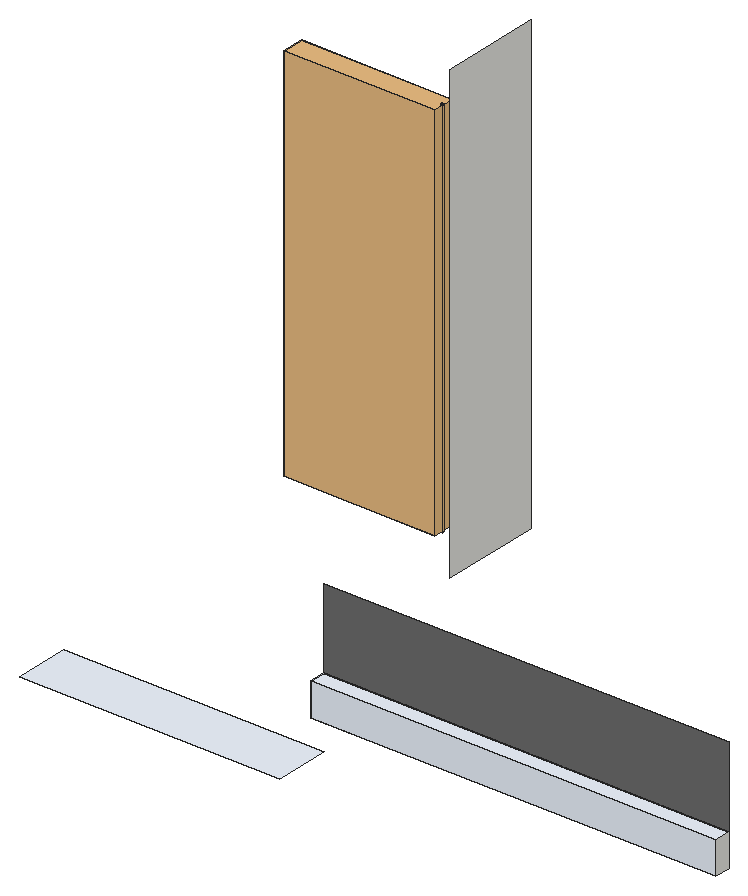
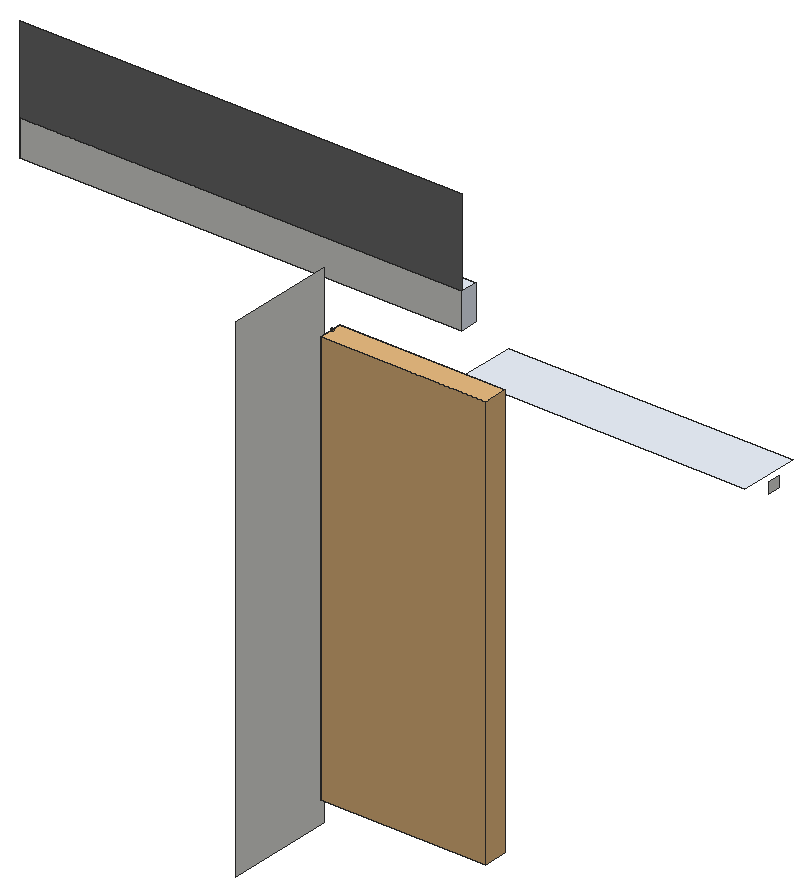
# SketchUp Ruby script. Lengths in inches.
U = 1.inch
M = Sketchup.active_model
def pt(a) = Geom::Point3d.new(a.map { |v| v * U })
def face(e, loops, mat)
  f = e.add_face(loops[0].map { |a| pt(a) })
  loops[1..].each { |l| e.add_face(l.map { |a| pt(a) }).erase! }
  f.material = f.back_material = mat if mat
  f
end
# faces: each face lists its corners as indices into pts; further lists are holes
def faces(e, pts, list, mat = nil) = list.each { |f| face(e, (f[0].is_a?(Array) ? f : [f]).map { |l| l.map { |i| pts[i] } }, mat) }
# xy, xz, yz: faces in a plane at the given z, y or x. An outline is a flat list of corners, or four numbers for a rectangle; further outlines are holes
def ring(l) = l.size == 4 ? [[l[0], l[1]], [l[2], l[1]], [l[2], l[3]], [l[0], l[3]]] : l.each_slice(2).to_a
def flat(e, list, mat, &to3) = list.each { |f| face(e, (f[0].is_a?(Array) ? f : [f]).map { |l| ring(l).map { |u, v| to3.(u, v) } }, mat) }
def xy(e, z, list, mat = nil) = flat(e, list, mat) { |x, y| [x, y, z] }
def xz(e, y, list, mat = nil) = flat(e, list, mat) { |x, z| [x, y, z] }
def yz(e, x, list, mat = nil) = flat(e, list, mat) { |y, z| [x, y, z] }
def lines(e, pts, list) = list.each { |a, b| e.add_line(pt(pts[a]), pt(pts[b])) }
# prism: a flat outline (further loops are holes) pulled along v
def prism(e, loops, v, mat = nil)
  f = face(e, loops, mat); d = Geom::Vector3d.new(v.map { |x| x * U })
  f.pushpull(f.normal.samedirection?(d) ? d.length : -d.length)
end
def box(e, o, s, mat = nil) = prism(e, [[o, [o[0] + s[0], o[1], o[2]], [o[0] + s[0], o[1] + s[1], o[2]], [o[0], o[1] + s[1], o[2]]]], [0, 0, s[2]], mat)
def at(x, y, z, deg = 0) = Geom::Transformation.translation(pt([x, y, z])) * Geom::Transformation.rotation(ORIGIN, Z_AXIS, deg.degrees)
def axes(o, x, y, z) = Geom::Transformation.new([*x, 0, *y, 0, *z, 0, *pt(o).to_a, 1])
def part(name) = M.definitions.add(name)
# library, detail: a bought-in or finely detailed component or shape, given as its bounding box
def library(name, o, s) = part(name).tap { |d| box(d.entities, o, s) }
def detail(e, o, s) = box(e.add_group.entities, o, s)
def put(e, d, t, mat = nil) = e.add_instance(d, t).tap { |i| i.material = mat if mat }
def group(e, t, mat = nil) = e.add_group.tap { |g| g.transformation = t; g.material = mat if mat }.entities
root = M.entities
M.materials.add("Generic").color = [111, 111, 111]
M.materials.add("Generic\#4").color = [238, 245, 255]
M.materials.add("Material \#1").color = [140, 140, 140]
c1 = library("3DGeom~6_Defintion",[-5.59,-471.8,-48.03],[468.87,1000,73.72])
c2 = library("3DGeom~9_Defintion",[456.52,-471.89,-18.89],[5.57,1000,5.49])
c3 = library("3DGeom~7_Defintion",[455.56,-471.94,-18.85],[5.55,1000,5.48])
c4 = part("3DGeom~8_Defintion")
xz(c4.entities,-471.94,[[458.125,-17.29,459.53,-16.11,457.73,-17.15],[458.125,-17.29,458.54,-17.29,459.53,-16.11],[458.54,-17.29,458.93,-17.15,459.53,-16.11],[457.73,-17.15,459.53,-16.11,457.42,-16.88],[458.93,-17.15,459.25,-16.88,459.53,-16.11],
  [457.42,-16.88,459.53,-16.11,457.21,-16.52],[459.25,-16.88,459.46,-16.52,459.53,-16.11],[457.21,-16.52,459.53,-16.11,457.14,-16.11],[457.14,-16.11,459.53,-16.11,457.21,-15.7],[459.53,-16.11,457.42,-15.34,457.21,-15.7],
  [459.53,-16.11,457.73,-15.07,457.42,-15.34],[459.53,-16.11,458.125,-14.93,457.73,-15.07],[459.53,-16.11,458.54,-14.93,458.125,-14.93],[459.53,-16.11,458.93,-15.07,458.54,-14.93],[459.53,-16.11,459.25,-15.34,458.93,-15.07],
  [459.53,-16.11,459.46,-15.7,459.25,-15.34]],"Material \#1")
xz(c4.entities,-416.39,[[458.125,-17.29,457.73,-17.15,459.53,-16.11],[458.125,-17.29,459.53,-16.11,458.54,-17.29],[458.54,-17.29,459.53,-16.11,458.93,-17.15],[457.73,-17.15,457.42,-16.88,459.53,-16.11],[458.93,-17.15,459.53,-16.11,459.25,-16.88],
  [457.42,-16.88,457.21,-16.52,459.53,-16.11],[459.25,-16.88,459.53,-16.11,459.46,-16.52],[457.21,-16.52,457.14,-16.11,459.53,-16.11],[457.14,-16.11,457.21,-15.7,459.53,-16.11],[459.53,-16.11,457.21,-15.7,457.42,-15.34],
  [459.53,-16.11,457.42,-15.34,457.73,-15.07],[459.53,-16.11,457.73,-15.07,458.125,-14.93],[459.53,-16.11,458.125,-14.93,458.54,-14.93],[459.53,-16.11,458.54,-14.93,458.93,-15.07],[459.53,-16.11,458.93,-15.07,459.25,-15.34],
  [459.53,-16.11,459.25,-15.34,459.46,-15.7]],"Material \#1")
xz(c4.entities,-27.5,[[458.125,-17.29,459.53,-16.11,457.73,-17.15],[458.125,-17.29,458.54,-17.29,459.53,-16.11],[458.54,-17.29,458.93,-17.15,459.53,-16.11],[457.73,-17.15,459.53,-16.11,457.42,-16.88],[458.93,-17.15,459.25,-16.88,459.53,-16.11],
  [457.42,-16.88,459.53,-16.11,457.21,-16.52],[459.25,-16.88,459.46,-16.52,459.53,-16.11],[457.21,-16.52,459.53,-16.11,457.14,-16.11],[457.14,-16.11,459.53,-16.11,457.21,-15.7],[459.53,-16.11,457.42,-15.34,457.21,-15.7],
  [459.53,-16.11,457.73,-15.07,457.42,-15.34],[459.53,-16.11,458.125,-14.93,457.73,-15.07],[459.53,-16.11,458.54,-14.93,458.125,-14.93],[459.53,-16.11,458.93,-15.07,458.54,-14.93],[459.53,-16.11,459.25,-15.34,458.93,-15.07],
  [459.53,-16.11,459.46,-15.7,459.25,-15.34]],"Material \#1")
xz(c4.entities,28.06,[[458.125,-17.29,457.73,-17.15,459.53,-16.11],[458.125,-17.29,459.53,-16.11,458.54,-17.29],[458.54,-17.29,459.53,-16.11,458.93,-17.15],[457.73,-17.15,457.42,-16.88,459.53,-16.11],[458.93,-17.15,459.53,-16.11,459.25,-16.88],
  [457.42,-16.88,457.21,-16.52,459.53,-16.11],[459.25,-16.88,459.53,-16.11,459.46,-16.52],[457.21,-16.52,457.14,-16.11,459.53,-16.11],[457.14,-16.11,457.21,-15.7,459.53,-16.11],[459.53,-16.11,457.21,-15.7,457.42,-15.34],
  [459.53,-16.11,457.42,-15.34,457.73,-15.07],[459.53,-16.11,457.73,-15.07,458.125,-14.93],[459.53,-16.11,458.125,-14.93,458.54,-14.93],[459.53,-16.11,458.54,-14.93,458.93,-15.07],[459.53,-16.11,458.93,-15.07,459.25,-15.34],
  [459.53,-16.11,459.25,-15.34,459.46,-15.7]],"Material \#1")
xz(c4.entities,472.5,[[458.125,-17.29,459.53,-16.11,457.73,-17.15],[458.125,-17.29,458.54,-17.29,459.53,-16.11],[458.54,-17.29,458.93,-17.15,459.53,-16.11],[457.73,-17.15,459.53,-16.11,457.42,-16.88],[458.93,-17.15,459.25,-16.88,459.53,-16.11],
  [457.42,-16.88,459.53,-16.11,457.21,-16.52],[459.25,-16.88,459.46,-16.52,459.53,-16.11],[457.21,-16.52,459.53,-16.11,457.14,-16.11],[457.14,-16.11,459.53,-16.11,457.21,-15.7],[459.53,-16.11,457.42,-15.34,457.21,-15.7],
  [459.53,-16.11,457.73,-15.07,457.42,-15.34],[459.53,-16.11,458.125,-14.93,457.73,-15.07],[459.53,-16.11,458.54,-14.93,458.125,-14.93],[459.53,-16.11,458.93,-15.07,458.54,-14.93],[459.53,-16.11,459.25,-15.34,458.93,-15.07],
  [459.53,-16.11,459.46,-15.7,459.25,-15.34]],"Material \#1")
xz(c4.entities,528.06,[[458.125,-17.29,457.73,-17.15,459.53,-16.11],[458.125,-17.29,459.53,-16.11,458.54,-17.29],[458.54,-17.29,459.53,-16.11,458.93,-17.15],[457.73,-17.15,457.42,-16.88,459.53,-16.11],[458.93,-17.15,459.53,-16.11,459.25,-16.88],
  [457.42,-16.88,457.21,-16.52,459.53,-16.11],[459.25,-16.88,459.53,-16.11,459.46,-16.52],[457.21,-16.52,457.14,-16.11,459.53,-16.11],[457.14,-16.11,457.21,-15.7,459.53,-16.11],[459.53,-16.11,457.21,-15.7,457.42,-15.34],
  [459.53,-16.11,457.42,-15.34,457.73,-15.07],[459.53,-16.11,457.73,-15.07,458.125,-14.93],[459.53,-16.11,458.125,-14.93,458.54,-14.93],[459.53,-16.11,458.54,-14.93,458.93,-15.07],[459.53,-16.11,458.93,-15.07,459.25,-15.34],
  [459.53,-16.11,459.25,-15.34,459.46,-15.7]],"Material \#1")
xy(root,162.6,[[128.43,116.3125,128.38,116.33,128.39,116.35],[128.43,116.3125,128.39,116.35,128.4375,116.33],[128.43,116.3125,128.4375,116.33,128.49,116.3125],[128.49,116.3125,128.4375,116.33,128.49,116.33],[128.49,116.3125,128.49,116.33,128.55,116.33],
  [128.38,116.33,128.34,116.37,128.35,116.375],[128.38,116.33,128.35,116.375,128.39,116.35],[128.49,116.33,128.54,116.35,128.55,116.33],[128.55,116.33,128.54,116.35,128.59,116.37],[128.54,116.35,128.58,116.375,128.59,116.37],
  [128.34,116.37,128.31,116.41,128.32,116.42],[128.34,116.37,128.32,116.42,128.35,116.375],[128.59,116.37,128.58,116.375,128.62,116.41],[128.58,116.375,128.6,116.42,128.62,116.41],[128.31,116.41,128.3,116.47,128.32,116.47],
  [128.31,116.41,128.32,116.47,128.32,116.42],[128.62,116.41,128.6,116.42,128.63,116.47],[128.6,116.42,128.61,116.47,128.63,116.47],[128.3,116.47,128.31,116.52,128.32,116.51],[128.3,116.47,128.32,116.51,128.32,116.47],
  [128.61,116.47,128.6,116.51,128.62,116.52],[128.61,116.47,128.62,116.52,128.63,116.47],[128.32,116.51,128.31,116.52,128.35,116.55],[128.6,116.51,128.58,116.55,128.59,116.5625],[128.6,116.51,128.59,116.5625,128.62,116.52],
  [128.31,116.52,128.34,116.5625,128.35,116.55],[128.35,116.55,128.34,116.5625,128.39,116.58],[128.58,116.55,128.54,116.58,128.55,116.6],[128.58,116.55,128.55,116.6,128.59,116.5625],[128.34,116.5625,128.38,116.6,128.39,116.58],
  [128.39,116.58,128.38,116.6,128.4375,116.6],[128.54,116.58,128.49,116.6,128.49,116.62],[128.54,116.58,128.49,116.62,128.55,116.6],[128.38,116.6,128.43,116.62,128.4375,116.6],[128.4375,116.6,128.43,116.62,128.49,116.6],
  [128.49,116.6,128.43,116.62,128.49,116.62]],"Material \#1")
xy(root,162.61,[[128.43,116.3125,128.4375,116.33,128.38,116.33],[128.43,116.3125,128.49,116.3125,128.49,116.33],[128.43,116.3125,128.49,116.33,128.4375,116.33],[128.49,116.3125,128.54,116.35,128.49,116.33],[128.49,116.3125,128.55,116.33,128.54,116.35],
  [128.38,116.33,128.39,116.35,128.34,116.37],[128.38,116.33,128.4375,116.33,128.39,116.35],[128.55,116.33,128.58,116.375,128.54,116.35],[128.55,116.33,128.59,116.37,128.58,116.375],[128.39,116.35,128.35,116.375,128.34,116.37],
  [128.34,116.37,128.35,116.375,128.31,116.41],[128.59,116.37,128.6,116.42,128.58,116.375],[128.59,116.37,128.62,116.41,128.6,116.42],[128.35,116.375,128.32,116.42,128.31,116.41],[128.31,116.41,128.32,116.42,128.3,116.47],
  [128.62,116.41,128.61,116.47,128.6,116.42],[128.62,116.41,128.63,116.47,128.61,116.47],[128.32,116.42,128.32,116.47,128.3,116.47],[128.3,116.47,128.32,116.47,128.31,116.52],[128.32,116.47,128.32,116.51,128.31,116.52],
  [128.61,116.47,128.63,116.47,128.6,116.51],[128.63,116.47,128.62,116.52,128.6,116.51],[128.32,116.51,128.34,116.5625,128.31,116.52],[128.32,116.51,128.35,116.55,128.34,116.5625],[128.6,116.51,128.62,116.52,128.58,116.55],
  [128.62,116.52,128.59,116.5625,128.58,116.55],[128.35,116.55,128.38,116.6,128.34,116.5625],[128.35,116.55,128.39,116.58,128.38,116.6],[128.58,116.55,128.59,116.5625,128.54,116.58],[128.59,116.5625,128.55,116.6,128.54,116.58],
  [128.39,116.58,128.43,116.62,128.38,116.6],[128.39,116.58,128.4375,116.6,128.43,116.62],[128.54,116.58,128.55,116.6,128.49,116.6],[128.4375,116.6,128.49,116.62,128.43,116.62],[128.4375,116.6,128.49,116.6,128.49,116.62],
  [128.49,116.6,128.55,116.6,128.49,116.62]],"Material \#1")
xy(root,166.09,[[128.43,116.3125,128.38,116.33,128.4375,116.33],[128.43,116.3125,128.4375,116.33,128.49,116.33],[128.43,116.3125,128.49,116.33,128.49,116.3125],[128.49,116.3125,128.49,116.33,128.54,116.35],[128.49,116.3125,128.54,116.35,128.55,116.33],
  [128.38,116.33,128.34,116.37,128.39,116.35],[128.38,116.33,128.39,116.35,128.4375,116.33],[128.55,116.33,128.54,116.35,128.58,116.375],[128.55,116.33,128.58,116.375,128.59,116.37],[128.39,116.35,128.34,116.37,128.35,116.375],
  [128.34,116.37,128.31,116.41,128.35,116.375],[128.59,116.37,128.58,116.375,128.6,116.42],[128.59,116.37,128.6,116.42,128.62,116.41],[128.35,116.375,128.31,116.41,128.32,116.42],[128.31,116.41,128.3,116.47,128.32,116.42],
  [128.62,116.41,128.6,116.42,128.61,116.47],[128.62,116.41,128.61,116.47,128.63,116.47],[128.32,116.42,128.3,116.47,128.32,116.47],[128.3,116.47,128.31,116.52,128.32,116.47],[128.32,116.47,128.31,116.52,128.32,116.51],
  [128.61,116.47,128.6,116.51,128.63,116.47],[128.63,116.47,128.6,116.51,128.62,116.52],[128.32,116.51,128.31,116.52,128.34,116.5625],[128.32,116.51,128.34,116.5625,128.35,116.55],[128.6,116.51,128.58,116.55,128.62,116.52],
  [128.62,116.52,128.58,116.55,128.59,116.5625],[128.35,116.55,128.34,116.5625,128.38,116.6],[128.35,116.55,128.38,116.6,128.39,116.58],[128.58,116.55,128.54,116.58,128.59,116.5625],[128.59,116.5625,128.54,116.58,128.55,116.6],
  [128.39,116.58,128.38,116.6,128.43,116.62],[128.39,116.58,128.43,116.62,128.4375,116.6],[128.54,116.58,128.49,116.6,128.55,116.6],[128.4375,116.6,128.43,116.62,128.49,116.62],[128.4375,116.6,128.49,116.62,128.49,116.6],
  [128.49,116.6,128.49,116.62,128.55,116.6]],"Material \#1")
xy(root,166.1,[[128.43,116.3125,128.39,116.35,128.38,116.33],[128.43,116.3125,128.4375,116.33,128.39,116.35],[128.43,116.3125,128.49,116.3125,128.4375,116.33],[128.49,116.3125,128.49,116.33,128.4375,116.33],[128.49,116.3125,128.55,116.33,128.49,116.33],
  [128.38,116.33,128.35,116.375,128.34,116.37],[128.38,116.33,128.39,116.35,128.35,116.375],[128.49,116.33,128.55,116.33,128.54,116.35],[128.55,116.33,128.59,116.37,128.54,116.35],[128.54,116.35,128.59,116.37,128.58,116.375],
  [128.34,116.37,128.32,116.42,128.31,116.41],[128.34,116.37,128.35,116.375,128.32,116.42],[128.59,116.37,128.62,116.41,128.58,116.375],[128.58,116.375,128.62,116.41,128.6,116.42],[128.31,116.41,128.32,116.47,128.3,116.47],
  [128.31,116.41,128.32,116.42,128.32,116.47],[128.62,116.41,128.63,116.47,128.6,116.42],[128.6,116.42,128.63,116.47,128.61,116.47],[128.3,116.47,128.32,116.47,128.32,116.51],[128.3,116.47,128.32,116.51,128.31,116.52],
  [128.61,116.47,128.62,116.52,128.6,116.51],[128.61,116.47,128.63,116.47,128.62,116.52],[128.32,116.51,128.35,116.55,128.31,116.52],[128.6,116.51,128.59,116.5625,128.58,116.55],[128.6,116.51,128.62,116.52,128.59,116.5625],
  [128.31,116.52,128.35,116.55,128.34,116.5625],[128.35,116.55,128.39,116.58,128.34,116.5625],[128.58,116.55,128.55,116.6,128.54,116.58],[128.58,116.55,128.59,116.5625,128.55,116.6],[128.34,116.5625,128.39,116.58,128.38,116.6],
  [128.39,116.58,128.4375,116.6,128.38,116.6],[128.54,116.58,128.49,116.62,128.49,116.6],[128.54,116.58,128.55,116.6,128.49,116.62],[128.38,116.6,128.4375,116.6,128.43,116.62],[128.4375,116.6,128.49,116.6,128.43,116.62],
  [128.49,116.6,128.49,116.62,128.43,116.62]],"Material \#1")
xy(root,175.6875,[[122.63,27.72,169.98,37.59]],"Generic\#4")
xy(root,182.625,[[169.98,34.65,243.69,37.59]],"Generic\#4")
xy(root,188.5625,[[169.98,34.65,243.69,37.59]],"Generic\#4")
xy(root,193.58,[[128.43,116.3125,128.38,116.33,128.39,116.35],[128.43,116.3125,128.39,116.35,128.4375,116.33],[128.43,116.3125,128.4375,116.33,128.49,116.3125],[128.49,116.3125,128.4375,116.33,128.49,116.33],[128.49,116.3125,128.49,116.33,128.55,116.33],
  [128.38,116.33,128.34,116.37,128.35,116.375],[128.38,116.33,128.35,116.375,128.39,116.35],[128.49,116.33,128.54,116.35,128.55,116.33],[128.55,116.33,128.54,116.35,128.59,116.37],[128.54,116.35,128.58,116.375,128.59,116.37],
  [128.34,116.37,128.31,116.41,128.32,116.42],[128.34,116.37,128.32,116.42,128.35,116.375],[128.59,116.37,128.58,116.375,128.62,116.41],[128.58,116.375,128.6,116.42,128.62,116.41],[128.31,116.41,128.3,116.47,128.32,116.47],
  [128.31,116.41,128.32,116.47,128.32,116.42],[128.62,116.41,128.6,116.42,128.63,116.47],[128.6,116.42,128.61,116.47,128.63,116.47],[128.3,116.47,128.31,116.52,128.32,116.51],[128.3,116.47,128.32,116.51,128.32,116.47],
  [128.61,116.47,128.6,116.51,128.62,116.52],[128.61,116.47,128.62,116.52,128.63,116.47],[128.32,116.51,128.31,116.52,128.35,116.55],[128.6,116.51,128.58,116.55,128.59,116.5625],[128.6,116.51,128.59,116.5625,128.62,116.52],
  [128.31,116.52,128.34,116.5625,128.35,116.55],[128.35,116.55,128.34,116.5625,128.39,116.58],[128.58,116.55,128.54,116.58,128.55,116.6],[128.58,116.55,128.55,116.6,128.59,116.5625],[128.34,116.5625,128.38,116.6,128.39,116.58],
  [128.39,116.58,128.38,116.6,128.4375,116.6],[128.54,116.58,128.49,116.6,128.49,116.62],[128.54,116.58,128.49,116.62,128.55,116.6],[128.38,116.6,128.43,116.62,128.4375,116.6],[128.4375,116.6,128.43,116.62,128.49,116.6],
  [128.49,116.6,128.43,116.62,128.49,116.62]],"Material \#1")
xy(root,193.6,[[128.43,116.3125,128.4375,116.33,128.38,116.33],[128.43,116.3125,128.49,116.3125,128.49,116.33],[128.43,116.3125,128.49,116.33,128.4375,116.33],[128.49,116.3125,128.54,116.35,128.49,116.33],[128.49,116.3125,128.55,116.33,128.54,116.35],
  [128.38,116.33,128.39,116.35,128.34,116.37],[128.38,116.33,128.4375,116.33,128.39,116.35],[128.55,116.33,128.58,116.375,128.54,116.35],[128.55,116.33,128.59,116.37,128.58,116.375],[128.39,116.35,128.35,116.375,128.34,116.37],
  [128.34,116.37,128.35,116.375,128.31,116.41],[128.59,116.37,128.6,116.42,128.58,116.375],[128.59,116.37,128.62,116.41,128.6,116.42],[128.35,116.375,128.32,116.42,128.31,116.41],[128.31,116.41,128.32,116.42,128.3,116.47],
  [128.62,116.41,128.61,116.47,128.6,116.42],[128.62,116.41,128.63,116.47,128.61,116.47],[128.32,116.42,128.32,116.47,128.3,116.47],[128.3,116.47,128.32,116.47,128.31,116.52],[128.32,116.47,128.32,116.51,128.31,116.52],
  [128.61,116.47,128.63,116.47,128.6,116.51],[128.63,116.47,128.62,116.52,128.6,116.51],[128.32,116.51,128.34,116.5625,128.31,116.52],[128.32,116.51,128.35,116.55,128.34,116.5625],[128.6,116.51,128.62,116.52,128.58,116.55],
  [128.62,116.52,128.59,116.5625,128.58,116.55],[128.35,116.55,128.38,116.6,128.34,116.5625],[128.35,116.55,128.39,116.58,128.38,116.6],[128.58,116.55,128.59,116.5625,128.54,116.58],[128.59,116.5625,128.55,116.6,128.54,116.58],
  [128.39,116.58,128.43,116.62,128.38,116.6],[128.39,116.58,128.4375,116.6,128.43,116.62],[128.54,116.58,128.55,116.6,128.49,116.6],[128.4375,116.6,128.49,116.62,128.43,116.62],[128.4375,116.6,128.49,116.6,128.49,116.62],
  [128.49,116.6,128.55,116.6,128.49,116.62]],"Material \#1")
xz(root,34.65,[[169.98,182.625,243.69,188.5625]],"Generic\#4")
xz(root,37.59,[[169.98,182.625,243.69,188.5625]])
xz(root,37.59,[[169.98,188.5625,243.69,203.1875]],"Generic")
yz(root,122.04,[[31.35,173.3125,33.48,175.125]])
yz(root,131.25,[[114.72,156.59,133.09,239.46]])
yz(root,169.98,[[34.65,182.625,37.59,188.5625]],"Generic\#4")
yz(root,243.69,[[34.65,182.625,37.59,188.5625]])
put(root,c1,axes([101.39,117.36,195.3125],[0.05875,0,0],[0,0,0.06934],[0,0.05495,0]),"Material \#1")
put(root,c2,axes([101.39,117.36,195.3125],[0.05894,0,0],[0,0,0.06956],[0,0.05513,0]),"Material \#1")
put(root,c3,axes([101.39,117.36,195.3125],[0.05906,0,0],[0,0,0.06971],[0,0.05524,0]),"Material \#1")
put(root,c4,axes([101.39,117.36,195.3125],[0.05906,0,0],[0,0,0.06971],[0,0.05524,0]),"Material \#1")
